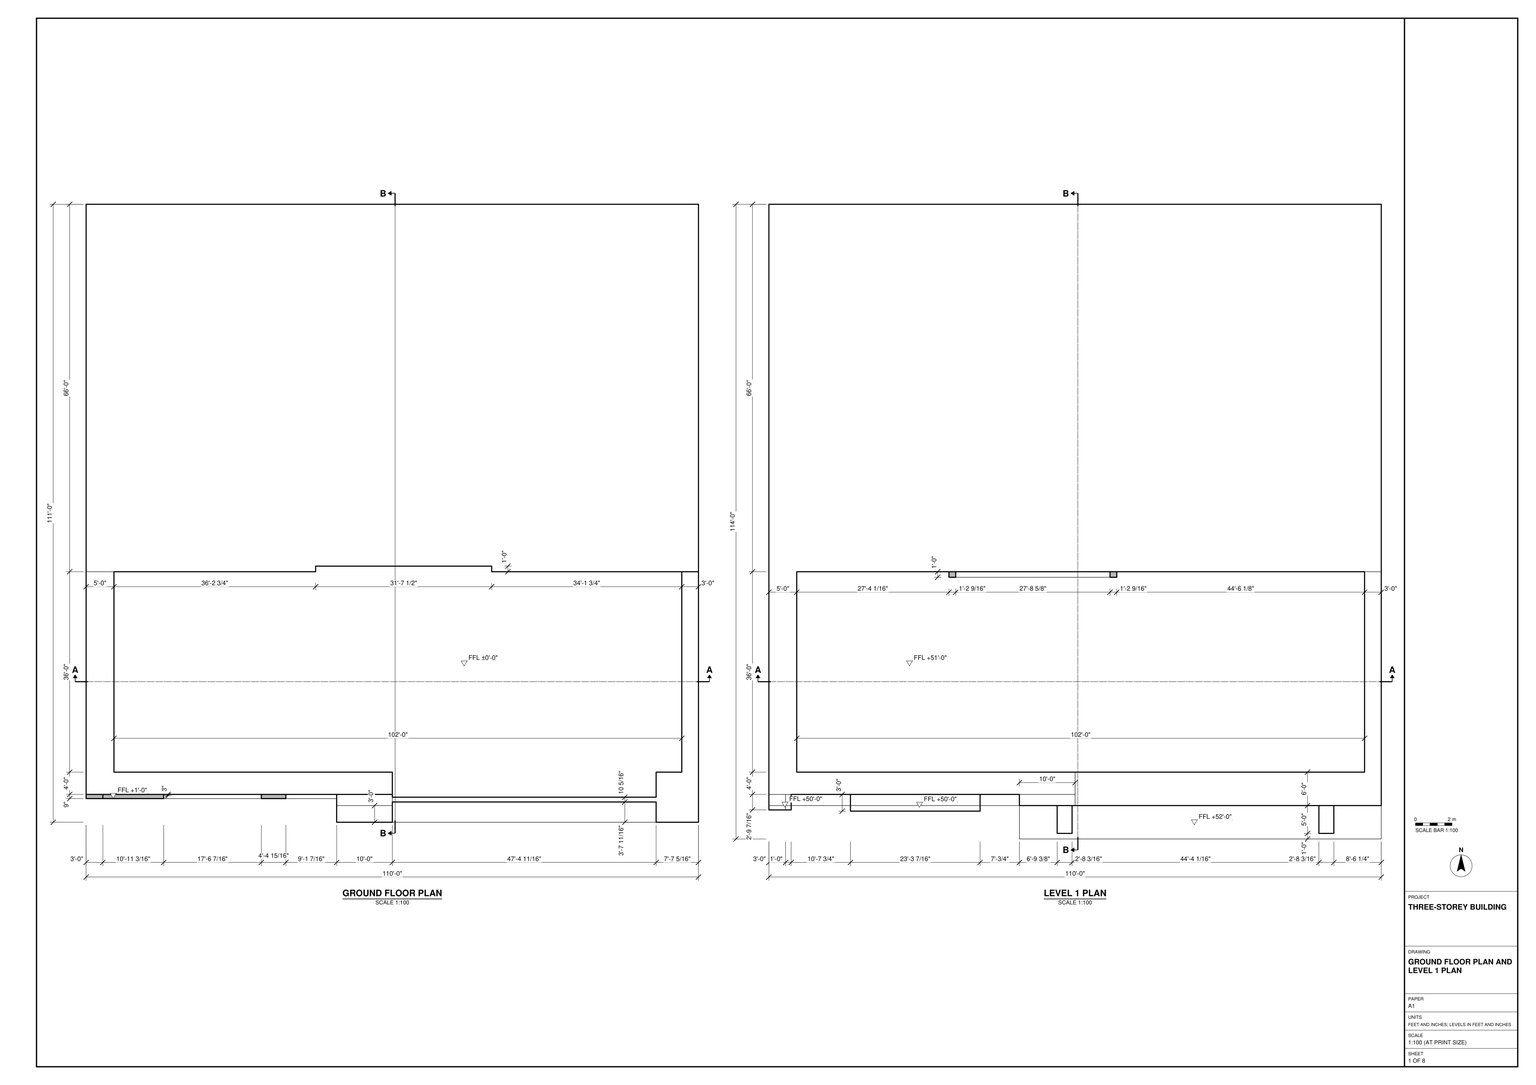
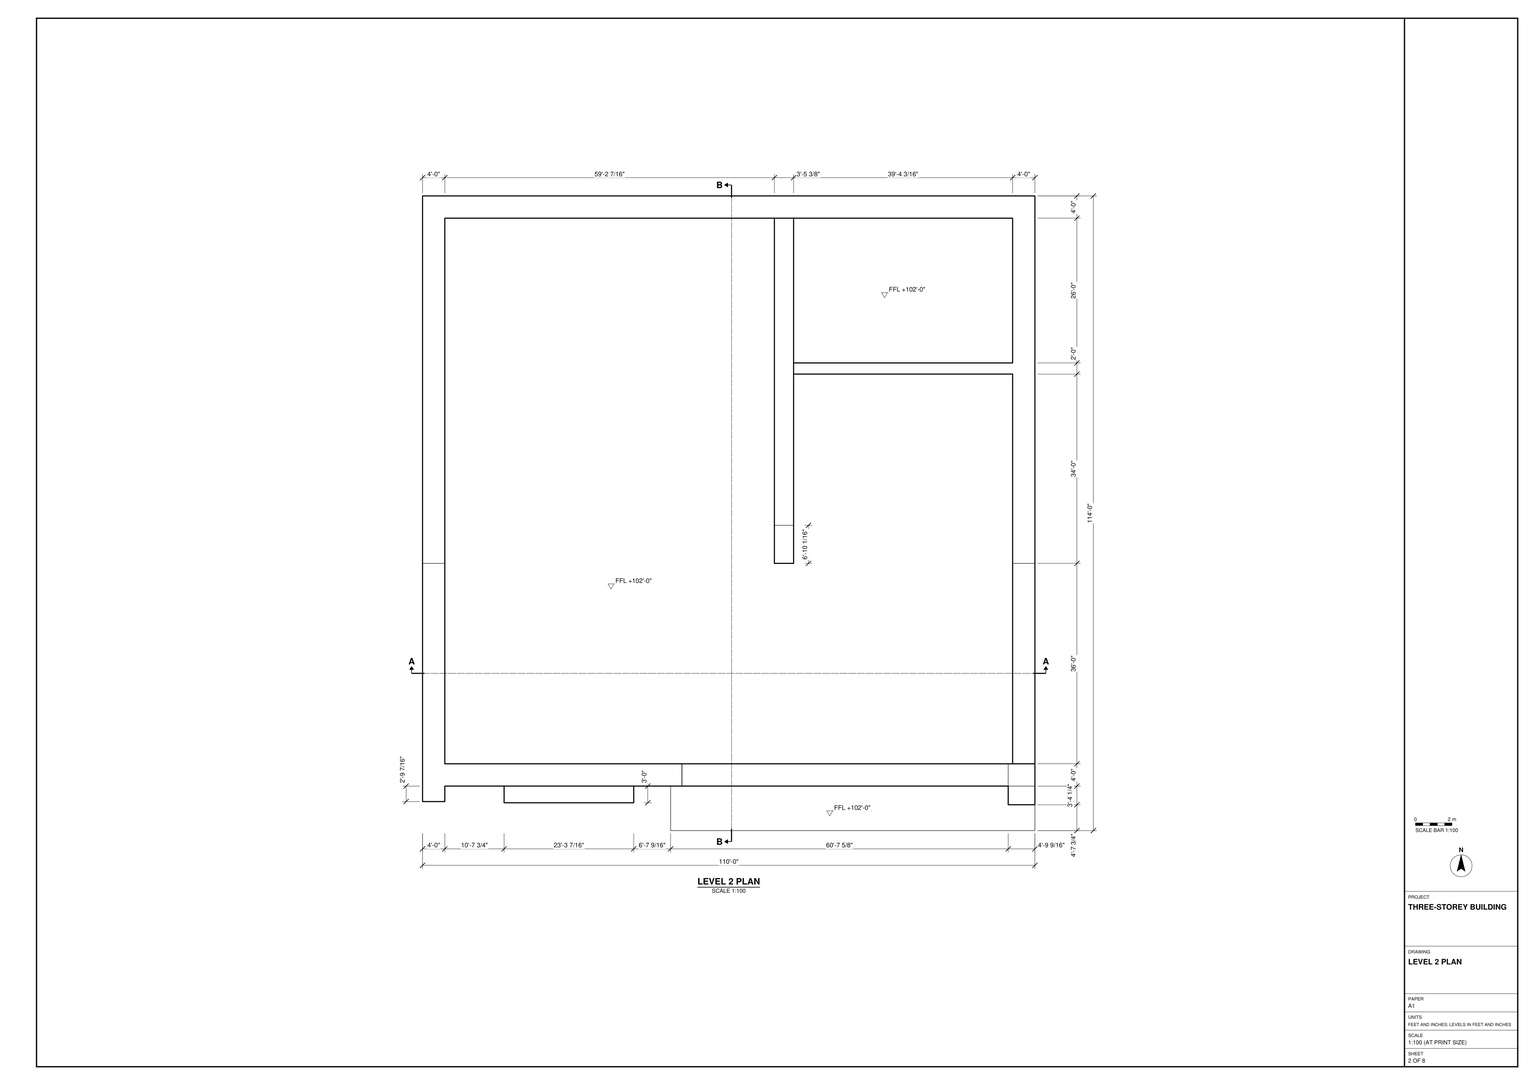
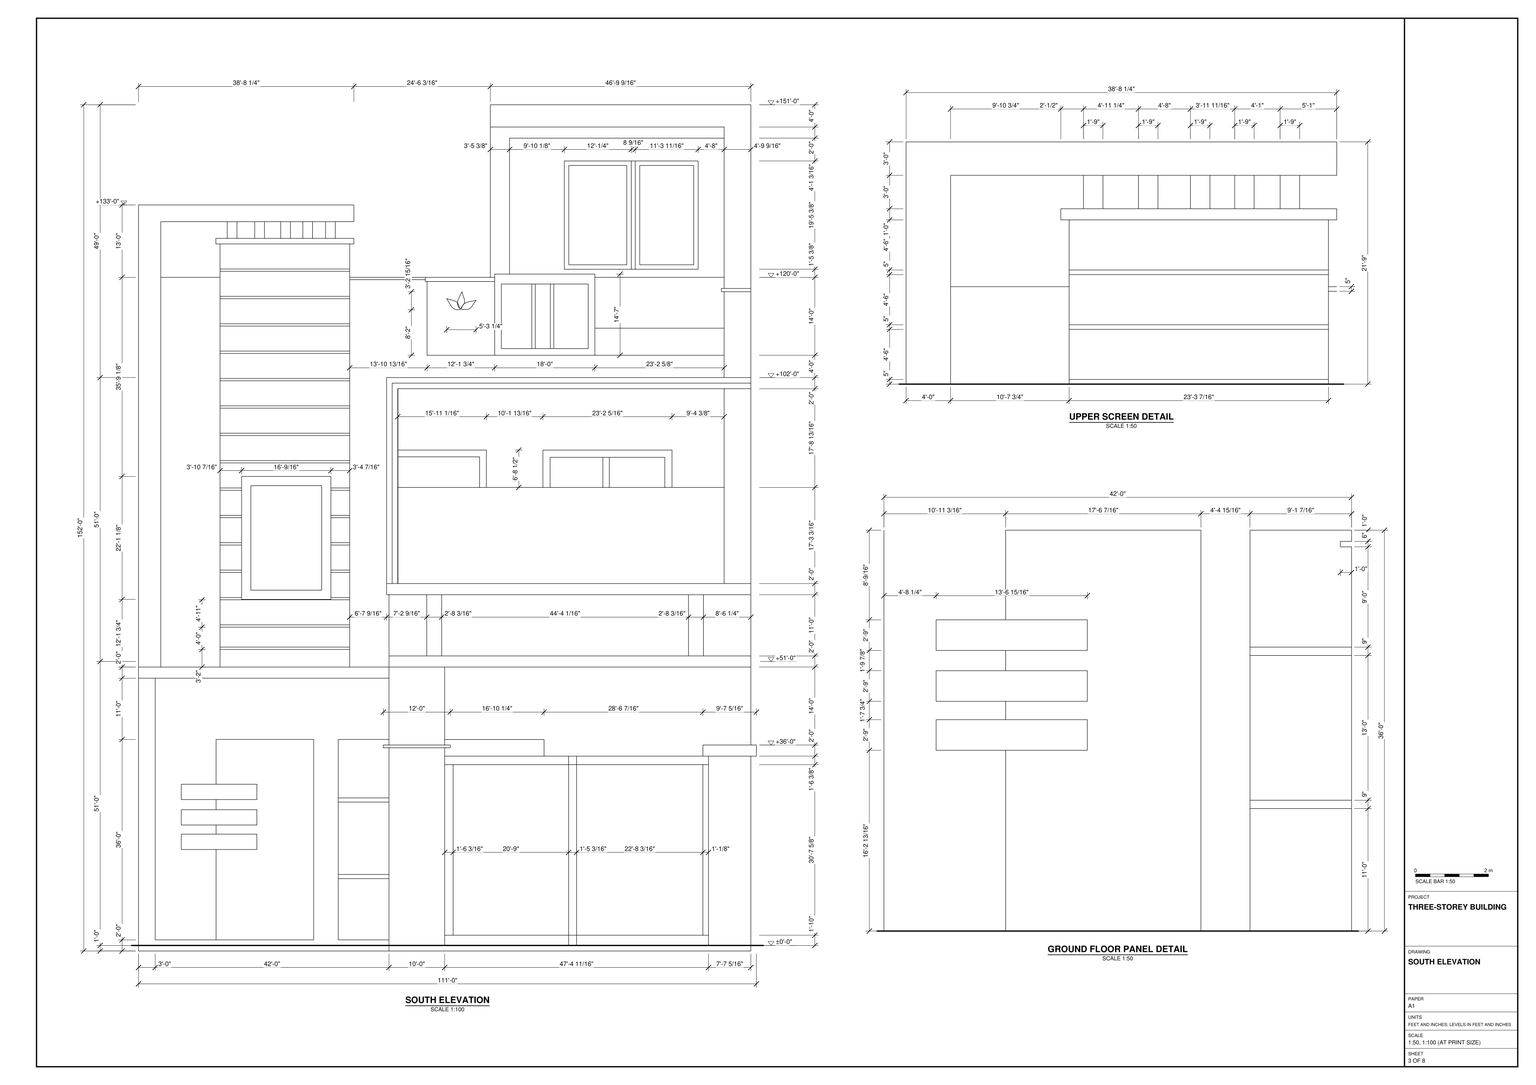
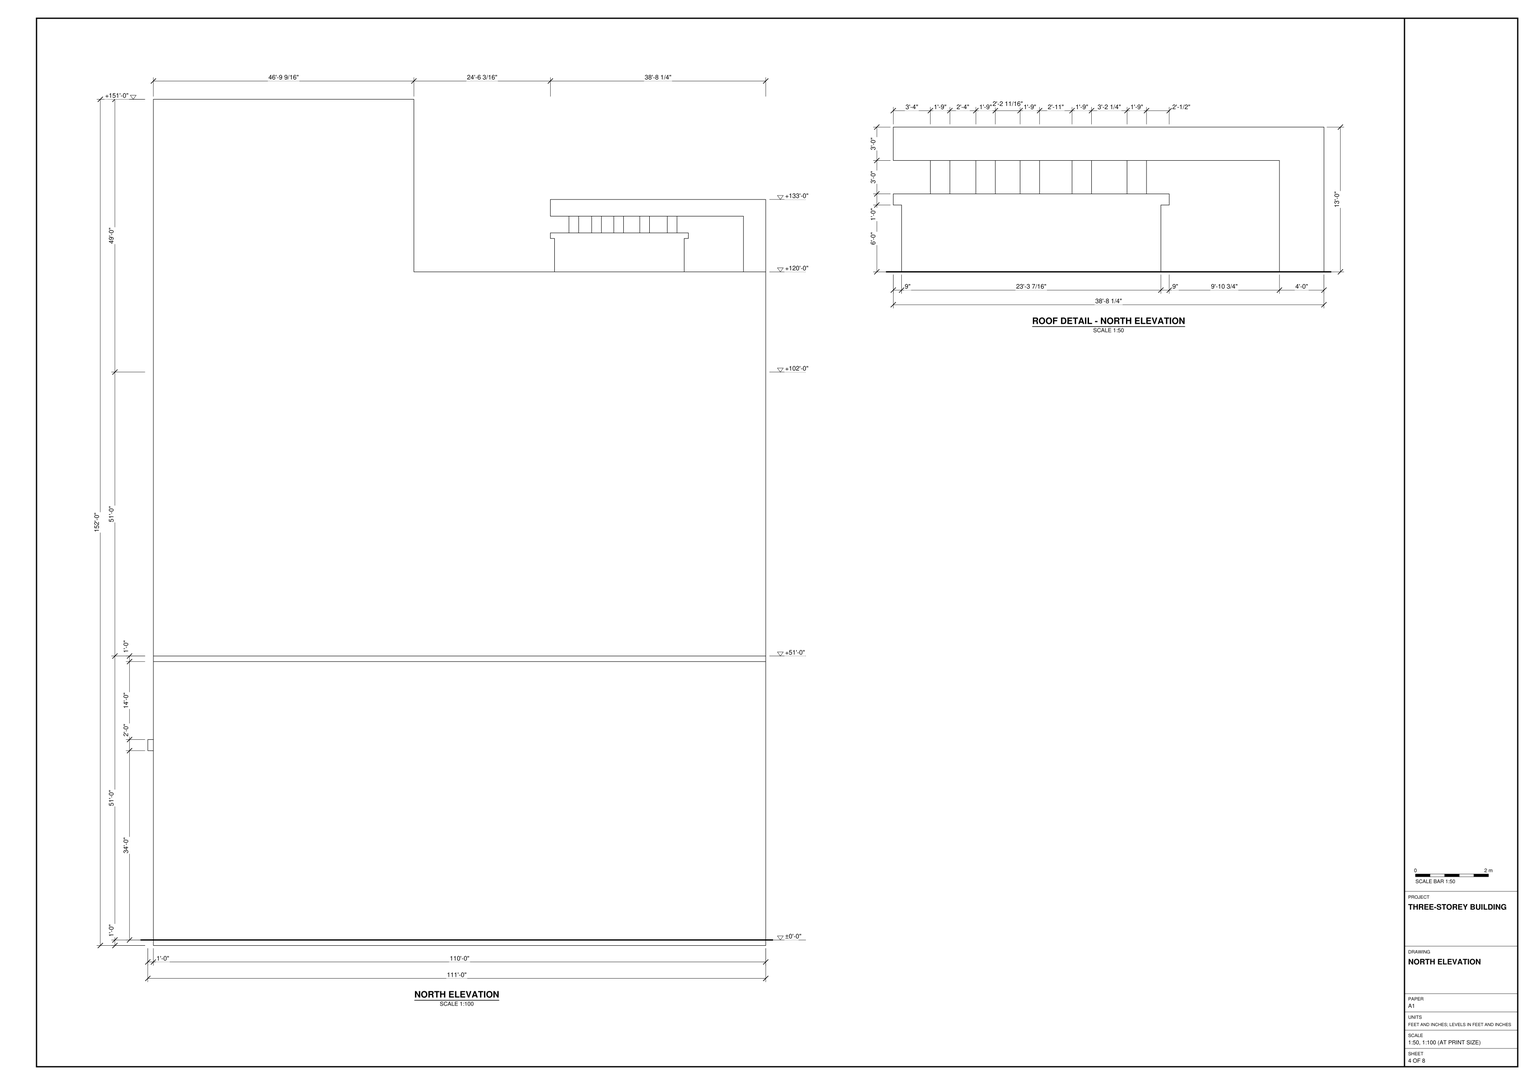
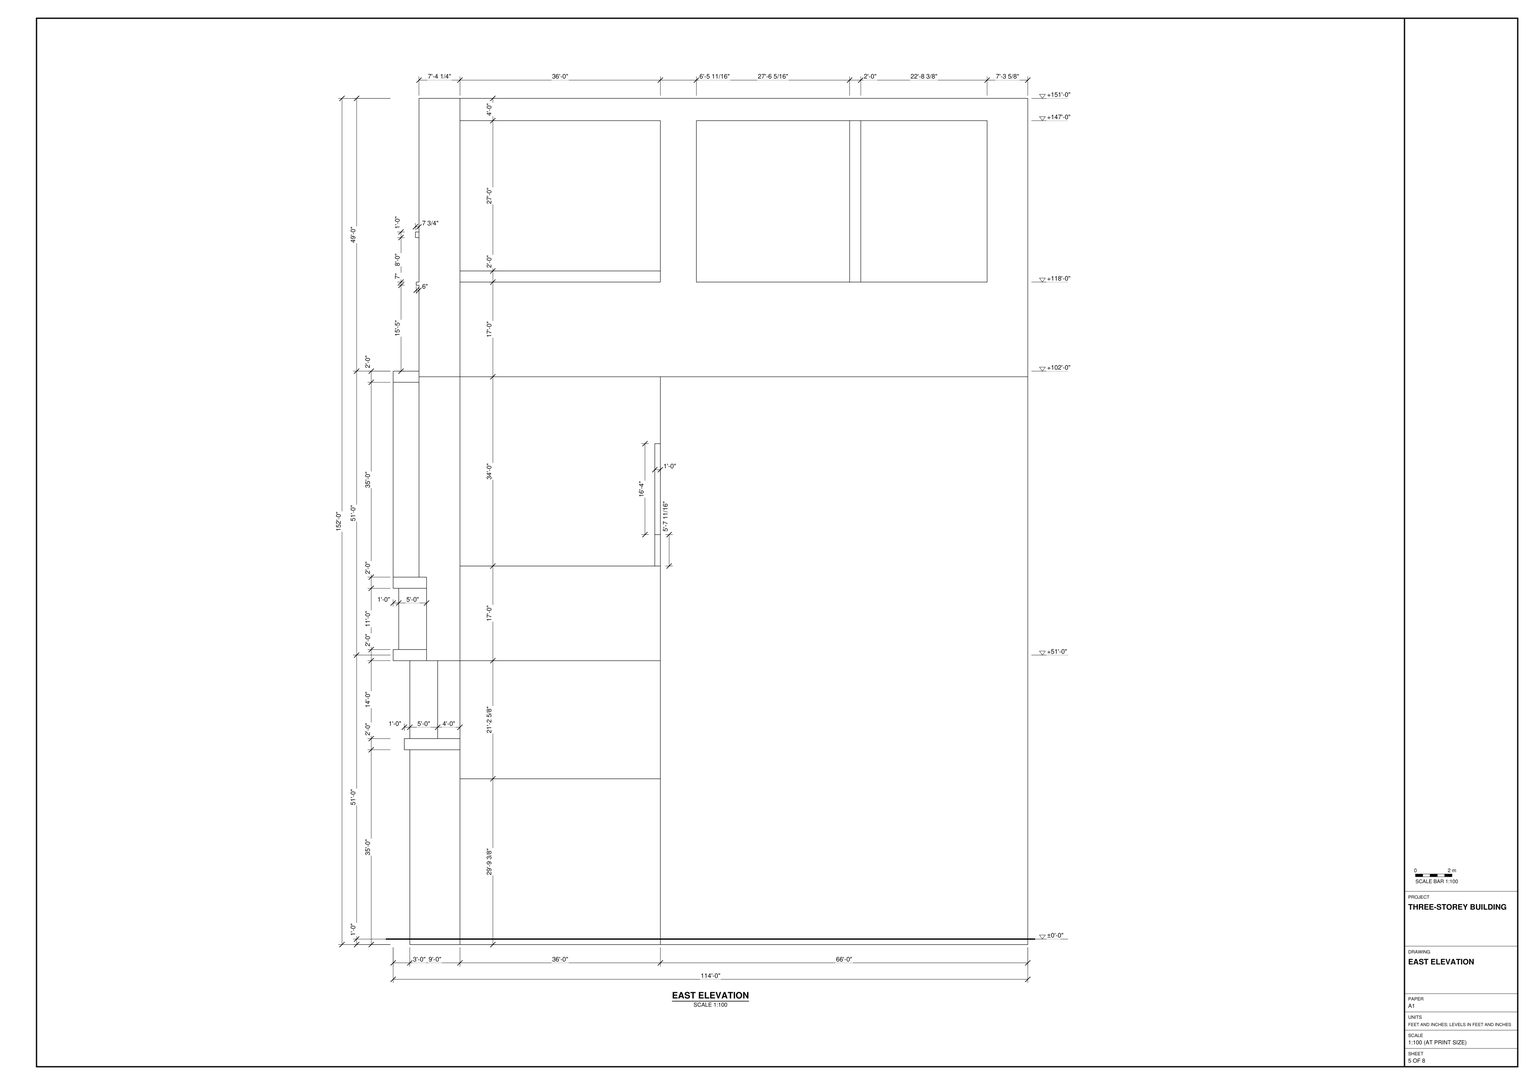
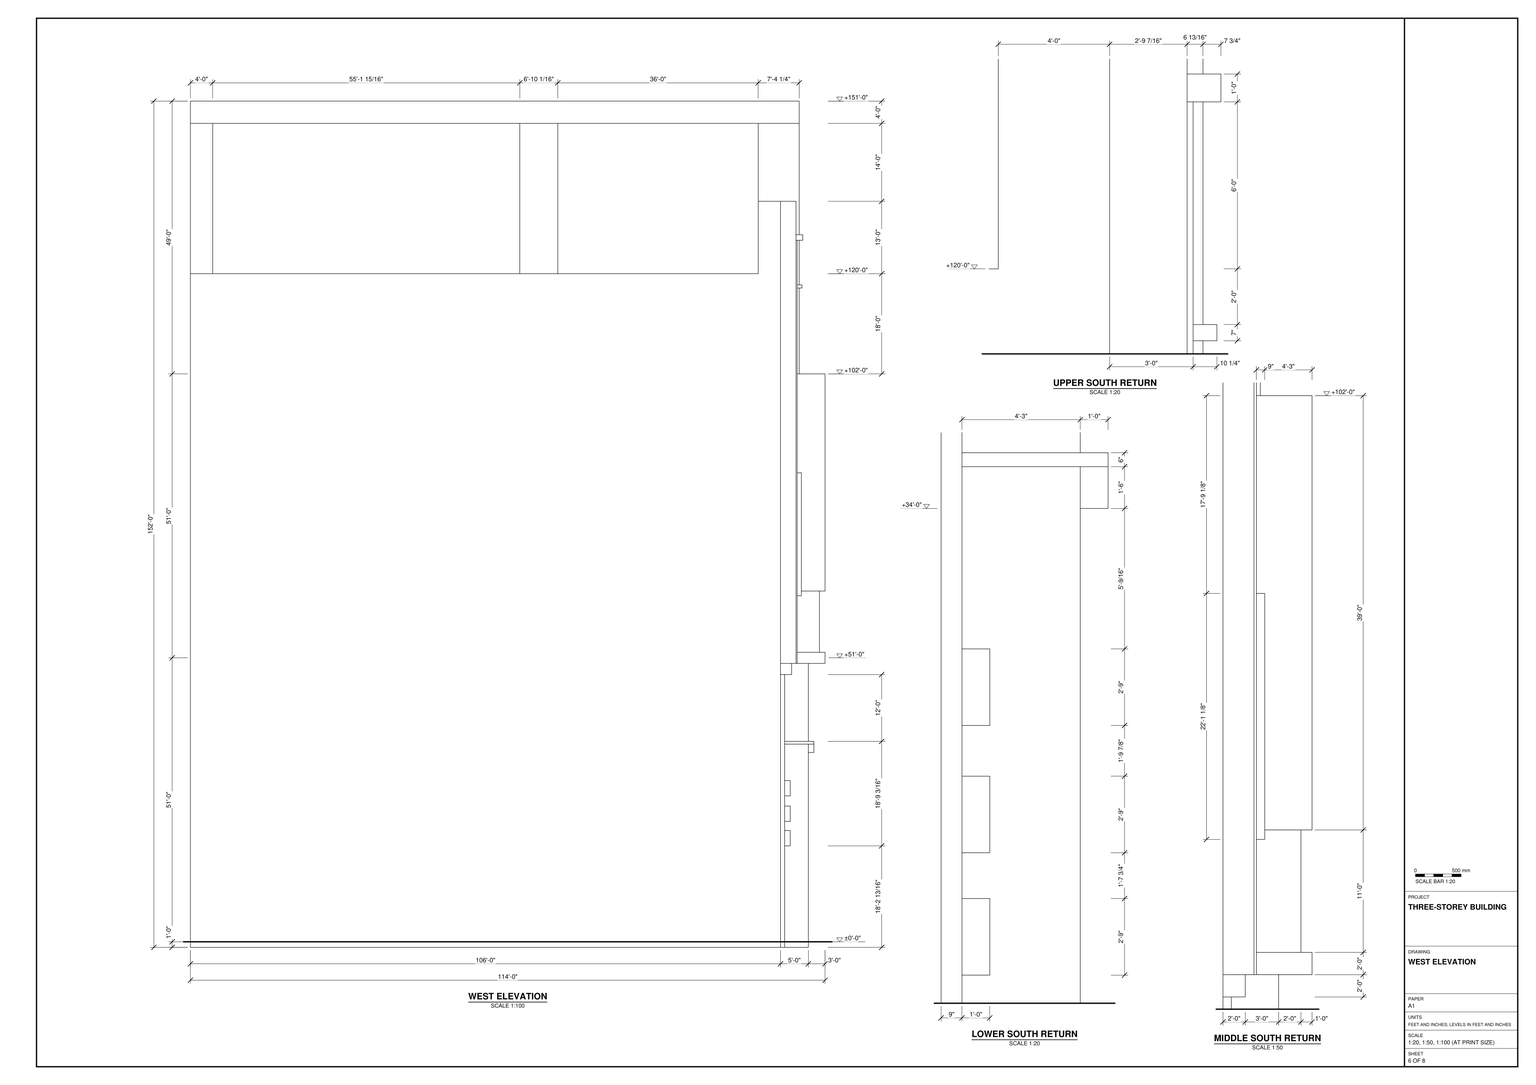
Build the three-storey building in SketchUp from task_files/diagram_01.pdf. Work in feet and inches. Set the overall model size to 111'-0" along X, 114'-0" along Y and 152'-0" along Z. Use finished floor levels of ±0'-0", +51'-0" and +102'-0".

Follow each floor plan for the slab outline, setbacks and projections along the south side. Model the walls at their drawn thicknesses. On the upper floor, place the internal wall and its cross wall so that the smaller space occupies the northeast corner. Use the elevations and sections to locate the openings, set the slab edges and form the stepped roofline. Include stairs, built-in joinery and main furniture where shown.

Use the enlarged south elevation details to model the three horizontal strips across the ground-floor panel and the banded screen above it. Keep the screen cap below the top of the taller bay to its right. Reproduce the broad middle-storey surround and the paired framed panels in the taller bay.

Keep shell elements such as walls, slabs and roof separate as groups or components. Group each furniture or joinery piece separately and use components for repeated parts. Any decor or loose items shown may be suitable library components. Save one SketchUp model as output_files/three_storey_building_with_a_stepped_south_facade.skp.

# SketchUp Ruby script. Lengths in inches.
U = 1.inch
M = Sketchup.active_model
def pt(a) = Geom::Point3d.new(a.map { |v| v * U })
def face(e, loops, mat)
  f = e.add_face(loops[0].map { |a| pt(a) })
  loops[1..].each { |l| e.add_face(l.map { |a| pt(a) }).erase! }
  f.material = f.back_material = mat if mat
  f
end
# faces: each face lists its corners as indices into pts; further lists are holes
def faces(e, pts, list, mat = nil) = list.each { |f| face(e, (f[0].is_a?(Array) ? f : [f]).map { |l| l.map { |i| pts[i] } }, mat) }
# xy, xz, yz: faces in a plane at the given z, y or x. An outline is a flat list of corners, or four numbers for a rectangle; further outlines are holes
def ring(l) = l.size == 4 ? [[l[0], l[1]], [l[2], l[1]], [l[2], l[3]], [l[0], l[3]]] : l.each_slice(2).to_a
def flat(e, list, mat, &to3) = list.each { |f| face(e, (f[0].is_a?(Array) ? f : [f]).map { |l| ring(l).map { |u, v| to3.(u, v) } }, mat) }
def xy(e, z, list, mat = nil) = flat(e, list, mat) { |x, y| [x, y, z] }
def xz(e, y, list, mat = nil) = flat(e, list, mat) { |x, z| [x, y, z] }
def yz(e, x, list, mat = nil) = flat(e, list, mat) { |y, z| [x, y, z] }
def lines(e, pts, list) = list.each { |a, b| e.add_line(pt(pts[a]), pt(pts[b])) }
# prism: a flat outline (further loops are holes) pulled along v
def prism(e, loops, v, mat = nil)
  f = face(e, loops, mat); d = Geom::Vector3d.new(v.map { |x| x * U })
  f.pushpull(f.normal.samedirection?(d) ? d.length : -d.length)
end
def box(e, o, s, mat = nil) = prism(e, [[o, [o[0] + s[0], o[1], o[2]], [o[0] + s[0], o[1] + s[1], o[2]], [o[0], o[1] + s[1], o[2]]]], [0, 0, s[2]], mat)
def at(x, y, z, deg = 0) = Geom::Transformation.translation(pt([x, y, z])) * Geom::Transformation.rotation(ORIGIN, Z_AXIS, deg.degrees)
def axes(o, x, y, z) = Geom::Transformation.new([*x, 0, *y, 0, *z, 0, *pt(o).to_a, 1])
def part(name) = M.definitions.add(name)
# library, detail: a bought-in or finely detailed component or shape, given as its bounding box
def library(name, o, s) = part(name).tap { |d| box(d.entities, o, s) }
def detail(e, o, s) = box(e.add_group.entities, o, s)
def put(e, d, t, mat = nil) = e.add_instance(d, t).tap { |i| i.material = mat if mat }
def group(e, t, mat = nil) = e.add_group.tap { |g| g.transformation = t; g.material = mat if mat }.entities
root = M.entities
M.materials.add("[0008_LavenderBlush]").color = [255, 240, 245]
M.materials.add("[0012_Bisque]").color = [153, 136, 117]
M.materials.add("[0022_Maroon]").color = [79, 0, 0]
M.materials.add("[0136_Charcoal]").color = [35, 35, 35]
M.materials.add("[0137_Black]").color = [0, 0, 0]
M.materials.add("[Blacktop Old 01]").color = [99, 102, 104]
M.materials.add("[Blacktop Old 01]1").color = [96, 99, 102]
M.materials.add("[Brick Basket]").color = [230, 156, 152]
M.materials.add("[Cladding Siding Tan]").color = [162, 126, 95]
M.materials.add("[Granite Brown]").color = [126, 104, 91]
M.materials.add("[Stone Flagstone Ashlar]").color = [175, 116, 102]
M.materials.add("[Stone Marble]").color = [143, 138, 136]
M.materials.add("[Translucent Glass Blue]").color = [74, 110, 175]
M.materials["[Translucent Glass Blue]"].alpha = 0.5
M.materials.add("[Translucent Resin Crush Gray]").color = [184, 184, 184]
M.materials["[Translucent Resin Crush Gray]"].alpha = 0.8
M.materials.add("[Wood Cherry Original]").color = [152, 86, 42]
xy(root,0,[[660,36,660,96,0,96,0,1368,1320,1368,1320,36],[540,36,660,72],[540,72,660,96],[0,87,540,96]])
xy(root,12,[[660,36,1228.6875,79.71]])
xy(root,12,[[660,90,1228.6875,90,1228.6875,144,1284,144,1284,576,874.23,576,874.23,588,494.73,588,494.73,576,60,576,60,144,660,144]],"[Stone Marble]")
xy(root,24,[[36,87,167.1875,93],[167.1875,87,377.625,96],[430.5625,87,540,96],[36,93,167.1875,96]])
xy(root,218.82,[[92.23,75,255.1875,87]])
xy(root,251.82,[[92.23,75,255.1875,87]])
xy(root,271.57,[[92.23,75,255.1875,87]])
xy(root,304.57,[[92.23,75,255.1875,87]])
xy(root,326.44,[[92.23,75,255.1875,87]])
xy(root,357.375,[[1284,144,1320,576]],"[Stone Flagstone Ashlar]")
xy(root,359.44,[[92.23,75,255.1875,87]])
xy(root,420,[[1320,36,1332,144],[660,79.71,1216.6875,90],[1216.6875,90,1228.6875,144]])
xy(root,420,[[1216.6875,24,1332,36],[1216.6875,36,1228.6875,79.71]],"[Stone Flagstone Ashlar]")
xy(root,438,[[528,24,672,36],[528,36,540,96],[660,36,672,96]],"[Stone Flagstone Ashlar]")
xy(root,444,[[528,24,672,24,672,96,660,96,660,36,540,36,540,96,528,96],[1216.6875,24,1332,144]],"[Stone Flagstone Ashlar]")
xy(root,455.8125,[[494.73,576,874.23,588]])
xy(root,456,[[167.1875,87,377.625,96],[430.5625,87,540,96]],"[Stone Flagstone Ashlar]")
xy(root,588,[[0,87,36,96],[36,87,540,96]])
xy(root,588,[[0,72,540,87]],"[Blacktop Old 01]")
xy(root,612,[[660,0,660,144,60,144,60,576,1320,576,1320,0],[540,36,660,72],[175.78,60,455.24,72],[0,62.58,36,72],[36,62.58,48,72],
  [0,72,36,96],[175.78,72,455.24,96],[540,72,660,96]])
xy(root,612,[[48,72,175.78,96],[455.24,72,540,96]],"[Blacktop Old 01]")
xy(root,612,[[540,0,660,36]],"[Brick Basket]")
xy(root,624,[[388.07,564,749.89,576]])
xy(root,624,[[60,144,1284,144,1284,576,749.89,576,749.89,564,388.07,564,388.07,576,60,576]],"[Stone Marble]")
xy(root,636,[[621.35,12,653.51,72],[1185.6,12,1217.76,72]])
xy(root,636,[[540,0,1320,0,1320,72,1217.76,72,1217.76,12,1185.6,12,1185.6,72,653.51,72,653.51,12,621.35,12,621.35,72,540,72]],"[Stone Flagstone Ashlar]")
xy(root,638.59,[[402.66,564,735.3,576]],"[Wood Cherry Original]")
xy(root,757.77,[[222.21,51,414.78,60],[222.21,60,414.78,96]])
xy(root,768,[[621.35,12,653.51,72],[1185.6,12,1217.76,72]])
xy(root,768,[[534.8125,0,534.8125,96,540,96,540,72,621.35,72,621.35,12,653.51,12,653.51,72,1185.6,72,1185.6,12,1217.76,12,1217.76,72,1320,72,1320,0]],"[Brick Basket]")
xy(root,777.71,[[242.15,51,394.84,96]])
xy(root,792,[[558.8125,96,558.875,144],[558.875,96,559.375,144]])
xy(root,792,[[558.8125,0,1320,0,1320,55.75,1262.44,55.75,1262.44,99.875,559.375,99.875,559.375,96,558.8125,96],[559.375,118.66,1262.44,144]],"[Stone Flagstone Ashlar]")
xy(root,816,[[1284,144,1320,576]],"[Stone Flagstone Ashlar]")
xy(root,883.7,[[871.73,564,1150.04,576]])
xy(root,899.27,[[887.3,564,1001.01,576],[1014.87,564,1134.47,576]],"[0136_Charcoal]")
xy(root,999.21,[[559.375,99.875,1262.44,118.66]])
xy(root,1002.96,[[242.15,51,394.84,96]])
xy(root,1022.9,[[222.21,51,414.78,60],[222.21,60,414.78,96]])
xy(root,1064.13,[[887.3,564,1001.01,576],[1014.87,564,1134.47,576]])
xy(root,1065.11,[[402.66,564,735.3,576]])
xy(root,1079.7,[[871.73,564,1150.04,576]])
xy(root,1079.7,[[388.07,564,749.89,576]],"[0022_Maroon]")
xy(root,1212,[[558.8125,0,558.8125,96,1262.44,96,1262.44,55.75,1320,55.75,1320,0]],"[Brick Basket]")
xy(root,1223.95,[[546.8125,0,600.6875,96]])
xy(root,1224,[[559.375,96,559.375,144,60,144,60,576,1320,576,1320,144,1262.44,144,1262.44,96],[558.8125,96,558.875,144],[558.875,96,559.375,144],[1262.44,96,1320,144]])
xy(root,1236,[[48,144,1272,144,1272,984,799.82,984,799.82,576,758.44,576,758.44,1320,48,1320],[758.44,658.04,799.82,1320],[799.82,1008,1272,1320]])
xy(root,1236,[[534.8125,0,1320,0,1320,55.75,1262.44,55.75,1262.44,96,534.8125,96]],"[Stone Flagstone Ashlar]")
xy(root,1284,[[767.8,84,983.8,96],[622.05,90,767.8,96]])
xy(root,1298.4,[[782.2,84,847.87,96],[847.87,84,855.29,96],[855.29,84,887.81,96],[887.81,84,895.23,96],[895.23,84,969.4,96]])
xy(root,1421.03,[[1256.44,49.75,1256.44,96,1262.44,96,1262.44,55.75,1320,55.75,1320,49.75]])
xy(root,1428,[[1256.44,49.75,1320,49.75,1320,55.75,1262.44,55.75,1262.44,96,1256.44,96],[1272,984,1320,1008],[1272,1008,1320,1280.39]])
xy(root,1428,[[1272,144,1320,576],[1272,653.67,1320,984]],"[Stone Flagstone Ashlar]")
xy(root,1437.6,[[782.2,84,847.87,96],[847.87,84,855.29,96],[855.29,84,887.81,96],[887.81,84,895.23,96],[895.23,84,969.4,96]])
xy(root,1443,[[618.05,84,767.8,90],[618.05,90,622.05,96]])
xy(root,1447,[[455.24,93,618.05,96]])
xy(root,1452,[[0,144,48,144,48,1320,758.44,1320,758.44,1368,0,1368]])
xy(root,1452,[[618.05,84,767.8,96],[455.24,93,618.05,93,618.05,96,1262.44,96,1262.44,144,48,144,48,96,455.24,96]],"[Stone Flagstone Ashlar]")
xy(root,1459,[[767.8,84,983.8,96]])
xy(root,1524,[[166.78,48,166.78,96,175.78,96,175.78,60,455.24,60,455.24,96,464.24,96,464.24,48]])
xy(root,1536,[[191.27,62.58,212.27,81.14],[250.52,62.58,271.52,81.14],[306.52,62.58,327.52,81.14],[354.21,62.58,375.21,81.14],[403.21,62.58,424.21,81.14]])
xy(root,1536,[[[166.78,48,464.24,96],[191.27,62.58,212.27,81.14],[250.52,62.58,271.52,81.14],[306.52,62.58,327.52,81.14],[354.21,62.58,375.21,81.14],[403.21,62.58,424.21,81.14]]],"[Brick Basket]")
xy(root,1572,[[48,62.58,48,144,464.24,144,464.24,62.58,424.21,62.58,424.21,81.14,403.21,81.14,403.21,62.58,375.21,62.58,375.21,81.14,354.21,81.14,354.21,62.58,327.52,62.58,327.52,81.14,306.52,81.14,306.52,62.58,271.52,62.58,271.52,81.14,250.52,81.14,250.52,62.58,212.27,62.58,212.27,81.14,191.27,81.14,191.27,62.58],[191.27,62.58,212.27,81.14],[250.52,62.58,271.52,81.14],[306.52,62.58,327.52,81.14],[354.21,62.58,375.21,81.14],
  [403.21,62.58,424.21,81.14]])
xy(root,1608,[[0,62.58,464.24,144]],"[Stone Flagstone Ashlar]")
xy(root,1752,[[799.82,576,1272,653.67]],"[Wood Cherry Original]")
xy(root,1775.95,[[758.44,653.67,799.82,658.04],[758.44,658.04,799.82,1320],[799.82,984,1272,1008]])
xy(root,1776,[[884.57,275.93,878.3,275.98,872.26,277.64,866.86,280.81,862.46,285.27,859.36,290.72,857.78,296.78,857.83,303.05,859.49,309.09,862.66,314.49,867.12,318.89,872.57,321.98,878.63,323.5625,884.9,323.52,890.9375,321.86,896.34,318.6875,900.74,314.23,903.84,308.78,905.42,302.72,905.37,296.45,903.71,290.41,900.54,285.01,896.08,280.61,890.63,277.51],[1154.19,275.93,1147.93,275.98,1141.89,277.64,1136.48,280.81,1132.08,285.27,1128.99,290.72,1127.41,296.78,1127.45,303.05,1129.12,309.09,1132.29,314.49,1136.75,318.89,1142.19,321.98,1148.26,323.5625,1154.52,323.52,1160.5625,321.86,1165.97,318.6875,1170.37,314.23,1173.46,308.78,1175.04,302.72,1175,296.45,1173.33,290.41,1170.16,285.01,1165.7,280.61,1160.26,277.51],[758.44,576,770.44,653.67],[770.44,576,1272,653.67],[1077.86,746.6,1071.59,746.64,1065.55,748.3,1060.15,751.47,1055.75,755.93,1052.65,761.38,1051.07,767.44,1051.12,773.71,1052.78,779.75,1055.95,785.15,1060.41,789.55,1065.86,792.65,1071.92,794.23,1078.18,794.18,1084.22,792.52,1089.63,789.35,1094.03,784.89,1097.125,779.44,1098.7,773.38,1098.66,767.11,1097,761.07,1093.83,755.67,1089.37,751.27,1083.92,748.17],
  [1272,984,1320,1008],[1272,1008,1320,1280.39]])
xy(root,1776,[[[758.44,55.75,758.44,576,1320,576,1320,144,1262.44,144,1262.44,55.75],[1154.19,275.93,1160.26,277.51,1165.7,280.61,1170.16,285.01,1173.33,290.41,1175,296.45,1175.04,302.72,1173.46,308.78,1170.37,314.23,1165.97,318.6875,1160.5625,321.86,1154.52,323.52,1148.26,323.5625,1142.19,321.98,1136.75,318.89,1132.29,314.49,1129.12,309.09,1127.45,303.05,1127.41,296.78,1128.99,290.72,1132.08,285.27,1136.48,280.81,1141.89,277.64,1147.93,275.98],[884.57,275.93,890.63,277.51,896.08,280.61,900.54,285.01,903.71,290.41,905.37,296.45,905.42,302.72,903.84,308.78,900.74,314.23,896.34,318.6875,890.9375,321.86,884.9,323.52,878.63,323.5625,872.57,321.98,867.12,318.89,862.66,314.49,859.49,309.09,857.83,303.05,857.78,296.78,859.36,290.72,862.46,285.27,866.86,280.81,872.26,277.64,878.3,275.98]],[[758.44,653.67,758.44,1320,1272,1320,1272,984,1320,984,1320,653.67],[1077.86,746.6,1083.92,748.17,1089.37,751.27,1093.83,755.67,1097,761.07,1098.66,767.11,1098.7,773.38,1097.125,779.44,1094.03,784.89,1089.63,789.35,1084.22,792.52,1078.18,794.18,1071.92,794.23,1065.86,792.65,1060.41,789.55,1055.95,785.15,1052.78,779.75,1051.12,773.71,1051.07,767.44,1052.65,761.38,1055.75,755.93,1060.15,751.47,1065.55,748.3,1071.59,746.64]]],"[Wood Cherry Original]")
xy(root,1824,[[758.44,55.75,1320,1368]])
xz(root,0,[[534.8125,768,1320,792]],"[Blacktop Old 01]")
xz(root,0,[[540,612,1320,636],[534.8125,792,546.8125,792,546.8125,1223.95,600.6875,1223.95,600.6875,1224,1320,1224,1320,1236,534.8125,1236],[546.8125,792,558.8125,792,558.8125,1212,1320,1212,1320,1224,600.6875,1224,600.6875,1223.95,546.8125,1223.95]],"[Stone Flagstone Ashlar]")
xz(root,12,[[621.35,636,653.51,768],[1185.6,636,1217.76,768]])
xz(root,24,[[1216.6875,420,1332,444],[528,438,672,444]],"[Stone Flagstone Ashlar]")
xz(root,36,[[540,0,1320,0,1320,420,1228.6875,420,1228.6875,12,660,12,660,438,540,438],[540,444,660,612]],"[Stone Flagstone Ashlar]")
xz(root,48,[[166.78,1524,464.24,1536]],"[Stone Flagstone Ashlar]")
xz(root,49.75,[[1256.44,1421.03,1320,1428]],"[Stone Flagstone Ashlar]")
xz(root,51,[[[222.21,757.77,414.78,1022.9],[242.15,777.71,394.84,1002.96]]])
xz(root,55.75,[[1262.44,792,1320,1212],[1262.44,1236,1320,1421.03],[1262.44,1428,1320,1428,1320,1824,758.44,1824,758.44,1776,1262.44,1776]],"[Stone Flagstone Ashlar]")
xz(root,60,[[175.78,650,455.24,655],[175.78,698,455.24,703],[175.78,757,455.24,757,455.24,762,414.78,762,414.78,757.77,222.21,757.77,222.21,762,175.78,762],[222.21,757.77,414.78,762],[175.78,816,222.21,821],
  [414.78,816,455.24,821],[175.78,875,222.21,880],[414.78,875,455.24,880],[175.78,934,222.21,939],[414.78,934,455.24,939],
  [175.78,993,222.21,998],[414.78,993,455.24,998],[175.78,1052,455.24,1057],[175.78,1111,455.24,1116],[175.78,1170,455.24,1175],
  [175.78,1229,455.24,1234],[175.78,1288,455.24,1293],[175.78,1347,455.24,1352],[175.78,1406,455.24,1411],[175.78,1465,455.24,1470]])
xz(root,60,[[175.78,612,455.24,650],[175.78,655,455.24,698],[175.78,703,455.24,757],[175.78,762,222.21,816],[414.78,762,455.24,816],
  [175.78,821,222.21,875],[414.78,821,455.24,875],[175.78,880,222.21,934],[414.78,880,455.24,934],[175.78,939,222.21,993],
  [414.78,939,455.24,993],[175.78,998,222.21,998,222.21,1022.9,414.78,1022.9,414.78,998,455.24,998,455.24,1052,175.78,1052],[175.78,1057,455.24,1111],[175.78,1116,455.24,1170],[175.78,1175,455.24,1229],
  [175.78,1234,455.24,1288],[175.78,1293,455.24,1347],[175.78,1352,455.24,1406],[175.78,1411,455.24,1465],[175.78,1470,455.24,1524]],"[Stone Flagstone Ashlar]")
xz(root,60,[[222.21,762,414.78,1022.9]],"[Translucent Glass Blue]")
xz(root,62.58,[[191.27,1536,212.27,1572],[250.52,1536,271.52,1572],[306.52,1536,327.52,1572],[354.21,1536,375.21,1572],[403.21,1536,424.21,1572]])
xz(root,62.58,[[0,612,48,612,48,1572,464.24,1572,464.24,1608,0,1608]],"[Stone Flagstone Ashlar]")
xz(root,72,[[621.35,636,653.51,768],[1185.6,636,1217.76,768]])
xz(root,72,[[0,588,540,612],[653.51,636,1185.6,768],[1217.76,636,1320,768]],"[Blacktop Old 01]")
xz(root,72,[[540,636,621.35,768]],"[Blacktop Old 01]1")
xz(root,75,[[92.23,218.82,255.1875,251.82],[92.23,271.57,255.1875,304.57],[92.23,326.44,255.1875,359.44]],"[Blacktop Old 01]")
xz(root,79.71,[[660,12,927.17,34.01],[927.17,12,944.34,34.01],[944.34,12,1228.6875,34.01],[660,34.01,678.2,401.64],[927.17,34.01,944.34,401.64],
  [1216.54,34.01,1228.6875,401.64],[660,401.64,927.17,420],[927.17,401.64,944.34,420],[944.34,401.64,1228.6875,420]],"[0137_Black]")
xz(root,79.71,[[678.2,34.01,927.17,401.64],[944.34,34.01,1216.54,401.64]],"[Cladding Siding Tan]")
xz(root,81.14,[[191.27,1536,212.27,1572],[250.52,1536,271.52,1572],[306.52,1536,327.52,1572],[354.21,1536,375.21,1572],[403.21,1536,424.21,1572]])
xz(root,84,[[[767.8,1284,983.8,1459],[782.2,1298.4,969.4,1437.6]],[847.87,1298.4,855.29,1437.6],[887.81,1298.4,895.23,1437.6]])
xz(root,84,[[618.05,1443,767.8,1452]],"[Stone Flagstone Ashlar]")
xz(root,87,[[92.23,218.82,167.1875,251.82],[167.1875,218.82,255.1875,251.82],[92.23,271.57,167.1875,304.57],[167.1875,271.57,255.1875,304.57],[167.1875,326.44,255.1875,359.44]])
xz(root,87,[[0,0,540,0,540,24,430.5625,24,430.5625,456,540,456,540,588,36,588,36,24,167.1875,24,167.1875,218.82,92.23,218.82,92.23,251.82,167.1875,251.82,167.1875,271.57,92.23,271.57,92.23,304.57,167.1875,304.57,167.1875,326.44,92.23,326.44,92.23,359.44,167.1875,359.44,167.1875,456,377.625,456,377.625,24,36,24,36,588,0,588]],"[Stone Flagstone Ashlar]")
xz(root,90,[[660,12,1228.6875,420],[688.6,1382.02,689.98,1382.2,693.6875,1383.22,692.68,1385.14,691.2,1386.45,690.29,1387.5,689.75,1388.74,689.07,1390.12,688.45,1391.32,688.04,1392.52,687.54,1393.72,687.4375,1394.9375,687.37,1396.15,687.5,1397.375,687.33,1397.57,686.34,1398.56,685.34,1399.26,684.01,1400.09,682.79,1400.55,680.85,1401.45,679.3125,1402,677.7,1402.33,676.37,1402.82,674.81,1403.09,673.55,1403.5,671.89,1403.85,670.62,1404.26,669.33,1404.54,667.99,1405.05,666.73,1405.35,665.66,1405.9,664.54,1406.36,665.89,1403.1,667.72,1400.63,669.71,1397.32,669.77,1396.65,670.625,1395.37,671.46,1394.15,672.1875,1393.14,672.87,1391.97,673.4375,1390.65,674.4,1389.63,675.18,1388.6,675.96,1387.59,676.85,1386.75,677.75,1385.95,678.8,1385.07,679.76,1384.29,680.8125,1383.69,681.89,1383.11,683.17,1382.87,684.4,1382.56,685.74,1382.42,687.27,1382.24],[696.42,1382.26,700.49,1382.875,703.55,1382.82,704.51,1382.84,706.33,1382.88,708.01,1382.87,709.43,1383,710.87,1383.15,712.06,1383.59,713.3125,1384.21,714.3,1384.93,715.52,1385.91,716.35,1386.92,717.84,1388.46,718.85,1389.74,719.69,1391.15,720.58,1392.25,721.35,1393.64,722.15,1394.7,723.02,1396.15,723.82,1397.22,724.51,1398.34,725.42,1399.44,726.12,1400.54,726.99,1401.37,727.79,1402.28,724.26,1402.07,721.33,1401.14,717.55,1400.34,716.91,1400.5,715.42,1400.1,713.99,1399.71,712.8,1399.35,711.47,1399.09,710.03,1398.98,708.76,1398.41,707.53,1398,706.32,1397.6,705.24,1397.02,704.1875,1396.44,703.01,1395.73,701.97,1395.07,701.53,1394.7,701.49,1394.625,700.72,1393.43,699.68,1392.11,698.59,1390.65,698.44,1390.45,698.25,1390.03,697.58,1388.64,696.93,1387.45,696.66,1386.09],[694.08,1383.9,696.09,1387.49,698.01,1389.875,698.44,1390.45,698.82,1391.25,699.51,1392.32,700.15,1393.44,701.05,1394.28,701.53,1394.7,702.25,1395.85,702.63,1397.06,702.92,1398.43,702.96,1399.66,702.92,1401.22,702.64,1402.5,702.34,1404.61,701.96,1406.2,701.36,1407.73,701.04,1409.11,700.41,1410.56,700.07,1411.84,699.45,1413.43,699.1,1414.71,698.64,1415.95,698.33,1417.35,697.89,1418.57,697.77,1419.76,697.55,1420.95,695.55,1418.04,694.48,1415.16,692.79,1411.68,692.27,1411.27,691.66,1409.86,691.1,1408.48,690.65,1407.33,690.04,1406.11,689.24,1404.92,688.91,1403.5625,688.48,1402.34,688.05,1401.14,687.84,1399.93,687.66,1398.74,687.5,1397.375,688.14,1396.6,688.75,1395.29,689.33,1393.99,689.87,1392.39,690.5,1390.6875,690.83,1389.78,691.78,1386.87,692.68,1385.14],[692.68,1385.14,691.78,1386.87,690.83,1389.78,690.5,1390.6875,689.87,1392.39,689.33,1393.99,688.75,1395.29,688.14,1396.6,687.5,1397.375,687.37,1396.15,687.4375,1394.9375,687.54,1393.72,688.04,1392.52,688.45,1391.32,689.07,1390.12,689.75,1388.74,690.29,1387.5,691.2,1386.45],
  [698.44,1390.45,698.59,1390.65,699.68,1392.11,700.72,1393.43,701.49,1394.625,701.53,1394.7,701.05,1394.28,700.15,1393.44,699.51,1392.32,698.82,1391.25]])
xz(root,90,[[[622.05,1284,767.8,1443],[688.6,1382.02,687.27,1382.24,685.74,1382.42,684.4,1382.56,683.17,1382.87,681.89,1383.11,680.8125,1383.69,679.76,1384.29,678.8,1385.07,677.75,1385.95,676.85,1386.75,675.96,1387.59,675.18,1388.6,674.4,1389.63,673.4375,1390.65,672.87,1391.97,672.1875,1393.14,671.46,1394.15,670.625,1395.37,669.77,1396.65,669.71,1397.32,667.72,1400.63,665.89,1403.1,664.54,1406.36,665.66,1405.9,666.73,1405.35,667.99,1405.05,669.33,1404.54,670.62,1404.26,671.89,1403.85,673.55,1403.5,674.81,1403.09,676.37,1402.82,677.7,1402.33,679.3125,1402,680.85,1401.45,682.79,1400.55,684.01,1400.09,685.34,1399.26,686.34,1398.56,687.33,1397.57,687.5,1397.375,688.14,1396.6,688.75,1395.29,689.33,1393.99,689.87,1392.39,690.5,1390.6875,690.83,1389.78,691.78,1386.87,692.68,1385.14,693.6875,1383.22,689.98,1382.2],[696.42,1382.26,696.66,1386.09,696.93,1387.45,697.58,1388.64,698.25,1390.03,698.44,1390.45,698.82,1391.25,699.51,1392.32,700.15,1393.44,701.05,1394.28,701.53,1394.7,701.97,1395.07,703.01,1395.73,704.1875,1396.44,705.24,1397.02,706.32,1397.6,707.53,1398,708.76,1398.41,710.03,1398.98,711.47,1399.09,712.8,1399.35,713.99,1399.71,715.42,1400.1,716.91,1400.5,717.55,1400.34,721.33,1401.14,724.26,1402.07,727.79,1402.28,726.99,1401.37,726.12,1400.54,725.42,1399.44,724.51,1398.34,723.82,1397.22,723.02,1396.15,722.15,1394.7,721.35,1393.64,720.58,1392.25,719.69,1391.15,718.85,1389.74,717.84,1388.46,716.35,1386.92,715.52,1385.91,714.3,1384.93,713.3125,1384.21,712.06,1383.59,710.87,1383.15,709.43,1383,708.01,1382.87,706.33,1382.88,704.51,1382.84,703.55,1382.82,700.49,1382.875],[694.08,1383.9,692.68,1385.14,691.2,1386.45,690.29,1387.5,689.75,1388.74,689.07,1390.12,688.45,1391.32,688.04,1392.52,687.54,1393.72,687.4375,1394.9375,687.37,1396.15,687.5,1397.375,687.66,1398.74,687.84,1399.93,688.05,1401.14,688.48,1402.34,688.91,1403.5625,689.24,1404.92,690.04,1406.11,690.65,1407.33,691.1,1408.48,691.66,1409.86,692.27,1411.27,692.79,1411.68,694.48,1415.16,695.55,1418.04,697.55,1420.95,697.77,1419.76,697.89,1418.57,698.33,1417.35,698.64,1415.95,699.1,1414.71,699.45,1413.43,700.07,1411.84,700.41,1410.56,701.04,1409.11,701.36,1407.73,701.96,1406.2,702.34,1404.61,702.64,1402.5,702.92,1401.22,702.96,1399.66,702.92,1398.43,702.63,1397.06,702.25,1395.85,701.53,1394.7,701.49,1394.625,700.72,1393.43,699.68,1392.11,698.59,1390.65,698.44,1390.45,698.01,1389.875,696.09,1387.49]]],"[Stone Flagstone Ashlar]")
xz(root,93,[[455.24,1447,618.05,1452]],"[Stone Flagstone Ashlar]")
xz(root,96,[[0,0,0,588,36,588,36,24,377.625,24,377.625,456,167.1875,456,167.1875,24,36,24,36,588,540,588,540,456,430.5625,456,430.5625,24,540,24,540,0],[540,0,540,438,528,438,528,444,540,444,540,612,660,612,660,0],[430.5625,156,540,165],[430.5625,321,540,330],[660,438,672,444],
  [0,588,540,612],[[175.78,612,455.24,1452],[222.21,757.77,414.78,1022.9]],[242.15,777.71,394.84,1002.96],[534.8125,792,546.8125,792,546.8125,1223.95,558.8125,1223.95,558.8125,1224,534.8125,1224],[546.8125,792,558.8125,1223.95],
  [558.8125,792,558.875,1212],[558.875,792,559.375,1212],[558.8125,1212,558.875,1223.95],[558.875,1212,559.375,1223.95],[559.375,1212,559.375,1223.95,600.6875,1223.95,600.6875,1224,1262.44,1224,1262.44,1212],
  [558.8125,1223.95,558.875,1224],[558.875,1223.95,559.375,1224],[559.375,1223.95,600.6875,1224],[534.8125,1224,1262.44,1236],[622.05,1284,622.05,1443,618.05,1443,618.05,1452,767.8,1452,767.8,1284],
  [[767.8,1284,983.8,1452],[782.2,1298.4,969.4,1437.6]],[847.87,1298.4,855.29,1437.6],[887.81,1298.4,895.23,1437.6],[767.8,1452,983.8,1459]])
xz(root,96,[[167.1875,24,377.625,456],[430.5625,24,540,156],[430.5625,165,540,321],[430.5625,330,540,330,540,438,528,438,528,444,540,444,540,456,430.5625,456],[48,612,175.78,1452],
  [455.24,612,540,612,540,768,534.8125,768,534.8125,1236,1262.44,1236,1262.44,1284,622.05,1284,622.05,1443,618.05,1443,618.05,1447,455.24,1447],[782.2,1298.4,847.87,1437.6],[855.29,1298.4,887.81,1437.6],[895.23,1298.4,969.4,1437.6]],"[Blacktop Old 01]")
xz(root,96,[[175.78,1452,175.78,1524,166.78,1524,166.78,1536,464.24,1536,464.24,1524,455.24,1524,455.24,1452]],"[Brick Basket]")
xz(root,96,[[983.8,1284,1262.44,1342.37],[983.8,1342.37,1262.44,1342.37,1262.44,1421.03,1256.44,1421.03,1256.44,1428,1262.44,1428,1262.44,1452,983.8,1452]],"[Stone Flagstone Ashlar]")
xz(root,99.875,[[559.375,792,1262.44,999.21]],"[Translucent Resin Crush Gray]")
xz(root,118.66,[[559.375,792,1262.44,999.21]])
xz(root,144,[[1228.6875,12,1228.6875,420,1216.6875,420,1216.6875,444,1284,444,1284,12],[1284,357.375,1284,444,1332,444,1332,420,1320,420,1320,357.375],[558.8125,792,558.875,1224],[558.875,792,559.375,1224],[1262.44,1224,1262.44,1236,1272,1236,1272,1428,1284,1428,1284,1224],
  [1284,1224,1320,1428],[48,1236,48,1452,1262.44,1452,1262.44,1428,1272,1428,1272,1236]])
xz(root,144,[[60,12,660,612],[60,624,60,1224,558.8125,1224,558.8125,792,1262.44,792,1262.44,624]],"[Granite Brown]")
xz(root,144,[[1262.44,624,1262.44,1224,1320,1224,1320,816,1284,816,1284,624],[1262.44,1428,1320,1776],[0,1452,0,1608,464.24,1608,464.24,1572,48,1572,48,1452]],"[Stone Flagstone Ashlar]")
xz(root,564,[[[388.07,624,749.89,1079.7],[402.66,638.59,735.3,1065.11]]],"[0022_Maroon]")
xz(root,564,[[[871.73,883.7,1150.04,1079.7],[887.3,899.27,1134.47,1064.13]],[1001.01,899.27,1014.87,1064.13]],"[0136_Charcoal]")
xz(root,576,[[1284,12,1320,357.375],[[388.07,624,749.89,1079.7],[402.66,638.59,735.3,1065.11]]])
xz(root,576,[[422.74,905.61,425.41,906.23,427.83,907.52,429.83,909.39,431.28,911.72,432.08,914.34,432.17,917.08,431.55,919.75,430.26,922.17,428.39,924.17,426.06,925.62,423.4375,926.42,420.7,926.51,418.03,925.89,415.61,924.6,413.61,922.73,412.16,920.4,411.36,917.78,411.27,915.04,411.89,912.37,413.18,909.95,415.05,907.95,417.375,906.5,420,905.7]],"[0008_LavenderBlush]")
xz(root,576,[[60,12,494.73,12,494.73,455.8125,874.23,455.8125,874.23,12,1284,12,1284,357.375,1320,357.375,1320,612,60,612],[[60,624,388.07,624,388.07,1079.7,749.89,1079.7,749.89,624,1284,624,1284,816,1320,816,1320,1224,60,1224],[871.73,883.7,1150.04,1079.7]]],"[Granite Brown]")
xz(root,576,[[758.44,1236,799.82,1236,799.82,1752,1272,1752,1272,1428,1320,1428,1320,1776,758.44,1776]],"[Stone Flagstone Ashlar]")
xz(root,576,[[887.3,899.27,1001.01,1064.13],[1014.87,899.27,1134.47,1064.13]],"[Translucent Glass Blue]")
xz(root,576,[[[402.66,638.59,735.3,1065.11],[422.74,905.61,420,905.7,417.375,906.5,415.05,907.95,413.18,909.95,411.89,912.37,411.27,915.04,411.36,917.78,412.16,920.4,413.61,922.73,415.61,924.6,418.03,925.89,420.7,926.51,423.4375,926.42,426.06,925.62,428.39,924.17,430.26,922.17,431.55,919.75,432.17,917.08,432.08,914.34,431.28,911.72,429.83,909.39,427.83,907.52,425.41,906.23]]],"[Wood Cherry Original]")
xz(root,588,[[519.87,307.91,524.84,308.57,529.47,310.49,533.45,313.54,536.5,317.51,538.42,322.14,539.07,327.11,538.42,332.08,536.5,336.71,533.45,340.69,529.47,343.74,524.84,345.66,519.87,346.3125,514.9,345.66,510.27,343.74,506.3,340.69,503.24,336.71,501.33,332.08,500.67,327.11,501.33,322.14,503.24,317.51,506.3,313.54,510.27,310.49,514.9,308.57]],"[0008_LavenderBlush]")
xz(root,588,[[[494.73,12,874.23,455.8125],[519.87,307.91,514.9,308.57,510.27,310.49,506.3,313.54,503.24,317.51,501.33,322.14,500.67,327.11,501.33,332.08,503.24,336.71,506.3,340.69,510.27,343.74,514.9,345.66,519.87,346.3125,524.84,345.66,529.47,343.74,533.45,340.69,536.5,336.71,538.42,332.08,539.07,327.11,538.42,322.14,536.5,317.51,533.45,313.54,529.47,310.49,524.84,308.57]]],"[Wood Cherry Original]")
xz(root,653.67,[[1272,1428,1272,1752,799.82,1752,799.82,1775.95,758.44,1775.95,758.44,1776,1320,1776,1320,1428]])
xz(root,984,[[[799.82,1236,1272,1775.95],[917.9375,1469.4,1206.4375,1702.8]],[1272,1428,1320,1776]],"[0012_Bisque]")
xz(root,984,[[[917.9375,1469.4,1062.1875,1702.8],[927.59,1479.06,1052.53,1693.15]],[1062.1875,1469.4,1070.75,1702.8],[[1070.75,1469.4,1206.4375,1702.8],[1080.4,1479.06,1196.78,1693.15]]],"[0137_Black]")
xz(root,984,[[927.59,1479.06,1052.53,1693.15],[1080.4,1479.06,1196.78,1693.15]],"[Translucent Glass Blue]")
xz(root,1008,[[799.82,1236,1272,1775.95]])
xz(root,1280.39,[[1272,1428,1320,1776]])
xz(root,1320,[[48,1236,758.44,1452],[758.44,1236,799.82,1775.95],[799.82,1236,1272,1236,1272,1776,758.44,1776,758.44,1775.95,799.82,1775.95]])
xz(root,1368,[[0,0,1320,12],[0,12,1320,612],[0,612,1320,624],[0,624,0,1452,758.44,1452,758.44,1824,1320,1824,1320,624]])
yz(root,0,[[96,0,96,1608,144,1608,144,1452,1368,1452,1368,0],[72,588,96,612]])
yz(root,0,[[87,0,96,588],[62.58,612,96,1608]],"[Stone Flagstone Ashlar]")
yz(root,36,[[87,24,93,588],[93,24,96,588]])
yz(root,48,[[144,1236,1320,1452]])
yz(root,48,[[62.58,612,96,612,96,1452,144,1452,144,1572,62.58,1572]],"[Stone Flagstone Ashlar]")
yz(root,60,[[144,12,576,612],[144,624,576,1224]],"[Granite Brown]")
yz(root,92.23,[[75,218.82,87,251.82],[75,271.57,87,304.57],[75,326.44,87,359.44]])
yz(root,166.78,[[48,1524,96,1536]],"[Stone Flagstone Ashlar]")
yz(root,167.1875,[[87,24,96,456]],"[Stone Flagstone Ashlar]")
yz(root,175.78,[[60,612,96,1524]],"[Stone Flagstone Ashlar]")
yz(root,191.27,[[62.58,1536,81.14,1572]])
yz(root,212.27,[[62.58,1536,81.14,1572]])
yz(root,222.21,[[51,757.77,60,1022.9],[60,757.77,96,1022.9]])
yz(root,242.15,[[51,777.71,96,1002.96]])
yz(root,250.52,[[62.58,1536,81.14,1572]])
yz(root,255.1875,[[75,218.82,87,251.82],[75,271.57,87,304.57],[75,326.44,87,359.44]])
yz(root,271.52,[[62.58,1536,81.14,1572]])
yz(root,306.52,[[62.58,1536,81.14,1572]])
yz(root,327.52,[[62.58,1536,81.14,1572]])
yz(root,354.21,[[62.58,1536,81.14,1572]])
yz(root,375.21,[[62.58,1536,81.14,1572]])
yz(root,377.625,[[87,24,96,456]],"[Stone Flagstone Ashlar]")
yz(root,388.07,[[564,624,576,1079.7]],"[0022_Maroon]")
yz(root,394.84,[[51,777.71,96,1002.96]])
yz(root,402.66,[[564,638.59,576,1065.11]],"[0022_Maroon]")
yz(root,403.21,[[62.58,1536,81.14,1572]])
yz(root,414.78,[[51,757.77,60,1022.9],[60,757.77,96,1022.9]])
yz(root,424.21,[[62.58,1536,81.14,1572]])
yz(root,430.5625,[[87,24,96,456]],"[Stone Flagstone Ashlar]")
yz(root,455.24,[[93,1447,96,1452]])
yz(root,455.24,[[60,612,96,612,96,1447,93,1447,93,1452,96,1452,96,1524,60,1524]],"[Stone Flagstone Ashlar]")
yz(root,464.24,[[48,1524,96,1536],[62.58,1572,144,1608]],"[Stone Flagstone Ashlar]")
yz(root,494.73,[[576,12,588,455.8125]])
yz(root,528,[[24,438,96,444]],"[Stone Flagstone Ashlar]")
yz(root,534.8125,[[0,768,96,1236]],"[Stone Flagstone Ashlar]")
yz(root,540,[[87,0,96,24],[87,456,96,588],[72,588,96,612],[72,636,96,768]])
yz(root,540,[[36,0,36,438,96,438,96,24,87,24,87,0],[36,444,36,612,72,612,72,588,87,588,87,456,96,456,96,444],[0,612,96,636]],"[Stone Flagstone Ashlar]")
yz(root,558.8125,[[96,792,144,1224]])
yz(root,558.8125,[[0,792,96,1212]],"[Stone Flagstone Ashlar]")
yz(root,558.875,[[96,792,144,1224]])
yz(root,559.375,[[96,792,99.875,792,99.875,999.21,118.66,999.21,118.66,792,144,792,144,1224,96,1224]],"[Granite Brown]")
yz(root,600.6875,[[0,1223.95,96,1224]])
yz(root,618.05,[[84,1443,84,1452,93,1452,93,1447,96,1447,96,1443],[93,1447,96,1452]])
yz(root,621.35,[[12,636,72,768]])
yz(root,622.05,[[90,1284,96,1443]])
yz(root,653.51,[[12,636,72,768]])
yz(root,660,[[96,12,144,612]],"[Granite Brown]")
yz(root,660,[[36,12,79.71,12,79.71,420,90,420,90,12,96,12,96,438,36,438],[36,444,96,612]],"[Stone Flagstone Ashlar]")
yz(root,672,[[24,438,96,444]],"[Stone Flagstone Ashlar]")
yz(root,735.3,[[564,638.59,576,1065.11]],"[Wood Cherry Original]")
yz(root,749.89,[[564,624,576,1079.7]],"[0022_Maroon]")
yz(root,758.44,[[576,1775.95,653.67,1776]])
yz(root,758.44,[[576,1236,658.04,1775.95],[658.04,1236,1320,1775.95],[1320,1452,1368,1776],[55.75,1776,1368,1824]],"[0012_Bisque]")
yz(root,767.8,[[84,1284,90,1443],[90,1284,90,1443,84,1443,84,1452,96,1452,96,1284],[84,1452,96,1459]])
yz(root,782.2,[[84,1298.4,96,1437.6]])
yz(root,799.82,[[984,1236,1008,1775.95],[1008,1236,1320,1775.95]])
yz(root,799.82,[[576,1236,984,1236,984,1775.95,653.67,1775.95,653.67,1752,576,1752]],"[0012_Bisque]")
yz(root,847.87,[[84,1298.4,96,1437.6]])
yz(root,855.29,[[84,1298.4,96,1437.6]])
yz(root,871.73,[[564,883.7,576,1079.7]])
yz(root,874.23,[[576,12,588,455.8125]])
yz(root,887.3,[[564,899.27,576,1064.13]],"[0136_Charcoal]")
yz(root,887.81,[[84,1298.4,96,1437.6]])
yz(root,895.23,[[84,1298.4,96,1437.6]])
yz(root,969.4,[[84,1298.4,96,1437.6]])
yz(root,983.8,[[84,1284,96,1459]])
yz(root,1001.01,[[564,899.27,576,1064.13]])
yz(root,1014.87,[[564,899.27,576,1064.13]])
yz(root,1134.47,[[564,899.27,576,1064.13]])
yz(root,1150.04,[[564,883.7,576,1079.7]])
yz(root,1185.6,[[12,636,72,768]])
yz(root,1216.6875,[[24,420,144,444]],"[Stone Flagstone Ashlar]")
yz(root,1217.76,[[12,636,72,768]])
yz(root,1228.6875,[[36,12,79.71,420],[90,12,144,420]],"[Stone Flagstone Ashlar]")
yz(root,1256.44,[[49.75,1421.03,96,1428]],"[Stone Flagstone Ashlar]")
yz(root,1262.44,[[55.75,792,55.75,1212,96,1212,96,1224,144,1224,144,792,118.66,792,118.66,999.21,99.875,999.21,99.875,792],[55.75,1236,96,1421.03],[55.75,1428,55.75,1776,144,1776,144,1452,96,1452,96,1428]],"[Stone Flagstone Ashlar]")
yz(root,1272,[[1008,1236,1008,1428,1280.39,1428,1280.39,1776,1320,1776,1320,1236],[984,1428,1008,1775.95],[1008,1428,1280.39,1776],[984,1775.95,1008,1776]])
yz(root,1272,[[144,1236,144,1428,576,1428,576,1752,653.67,1752,653.67,1428,984,1428,984,1236]],"[Stone Flagstone Ashlar]")
yz(root,1284,[[144,12,576,357.375],[144,624,576,816]],"[Stone Flagstone Ashlar]")
yz(root,1320,[[576,0,1368,12],[576,12,1368,1224],[[144,1224,1368,1224,1368,1824,144,1824,144,1776,576,1776,576,1428,144,1428],[653.67,1428,1280.39,1776]],[984,1428,1008,1776],[1008,1428,1280.39,1776]])
yz(root,1320,[[36,0,144,420],[144,0,576,357.375],[0,612,72,636],[72,612,144,612,144,1224,55.75,1224,55.75,792,72,792],[144,612,576,816],
  [0,768,72,792],[0,1212,55.75,1236],[55.75,1224,144,1224,144,1824,55.75,1824,55.75,1428,49.75,1428,49.75,1421.03,55.75,1421.03]],"[Stone Flagstone Ashlar]")
yz(root,1332,[[24,420,144,444]],"[Stone Flagstone Ashlar]")
# 10 loose lines left out
